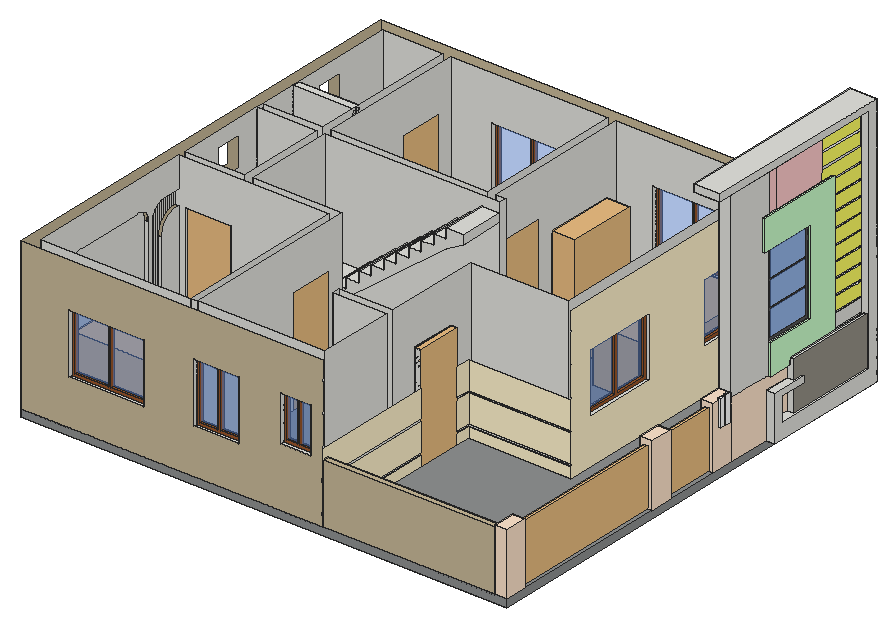
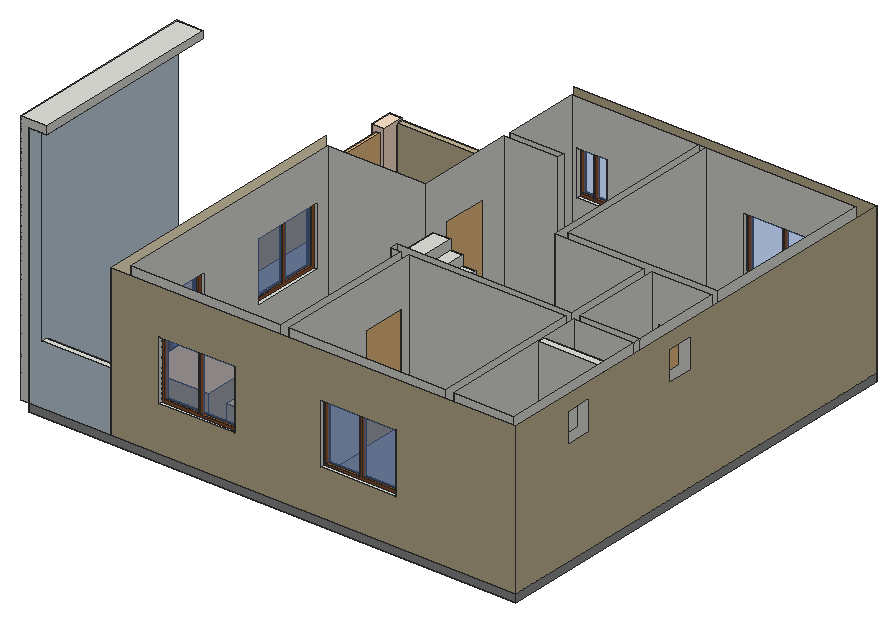
# SketchUp Ruby script. Lengths in inches.
U = 1.inch
M = Sketchup.active_model
def pt(a) = Geom::Point3d.new(a.map { |v| v * U })
def face(e, loops, mat)
  f = e.add_face(loops[0].map { |a| pt(a) })
  loops[1..].each { |l| e.add_face(l.map { |a| pt(a) }).erase! }
  f.material = f.back_material = mat if mat
  f
end
# faces: each face lists its corners as indices into pts; further lists are holes
def faces(e, pts, list, mat = nil) = list.each { |f| face(e, (f[0].is_a?(Array) ? f : [f]).map { |l| l.map { |i| pts[i] } }, mat) }
# xy, xz, yz: faces in a plane at the given z, y or x. An outline is a flat list of corners, or four numbers for a rectangle; further outlines are holes
def ring(l) = l.size == 4 ? [[l[0], l[1]], [l[2], l[1]], [l[2], l[3]], [l[0], l[3]]] : l.each_slice(2).to_a
def flat(e, list, mat, &to3) = list.each { |f| face(e, (f[0].is_a?(Array) ? f : [f]).map { |l| ring(l).map { |u, v| to3.(u, v) } }, mat) }
def xy(e, z, list, mat = nil) = flat(e, list, mat) { |x, y| [x, y, z] }
def xz(e, y, list, mat = nil) = flat(e, list, mat) { |x, z| [x, y, z] }
def yz(e, x, list, mat = nil) = flat(e, list, mat) { |y, z| [x, y, z] }
def lines(e, pts, list) = list.each { |a, b| e.add_line(pt(pts[a]), pt(pts[b])) }
# prism: a flat outline (further loops are holes) pulled along v
def prism(e, loops, v, mat = nil)
  f = face(e, loops, mat); d = Geom::Vector3d.new(v.map { |x| x * U })
  f.pushpull(f.normal.samedirection?(d) ? d.length : -d.length)
end
def box(e, o, s, mat = nil) = prism(e, [[o, [o[0] + s[0], o[1], o[2]], [o[0] + s[0], o[1] + s[1], o[2]], [o[0], o[1] + s[1], o[2]]]], [0, 0, s[2]], mat)
def at(x, y, z, deg = 0) = Geom::Transformation.translation(pt([x, y, z])) * Geom::Transformation.rotation(ORIGIN, Z_AXIS, deg.degrees)
def axes(o, x, y, z) = Geom::Transformation.new([*x, 0, *y, 0, *z, 0, *pt(o).to_a, 1])
def part(name) = M.definitions.add(name)
# library, detail: a bought-in or finely detailed component or shape, given as its bounding box
def library(name, o, s) = part(name).tap { |d| box(d.entities, o, s) }
def detail(e, o, s) = box(e.add_group.entities, o, s)
def put(e, d, t, mat = nil) = e.add_instance(d, t).tap { |i| i.material = mat if mat }
def group(e, t, mat = nil) = e.add_group.tap { |g| g.transformation = t; g.material = mat if mat }.entities
root = M.entities
M.materials.add("[Blacktop Old 02]").color = [143, 145, 145]
M.materials.add("[Color A01]").color = [255, 204, 204]
M.materials.add("[Color C01]").color = [255, 229, 204]
M.materials.add("[Color D01]").color = [255, 242, 204]
M.materials.add("[Color E03]").color = [255, 255, 101]
M.materials.add("[Color F02]").color = [204, 255, 153]
M.materials.add("[Color G01]").color = [204, 255, 204]
M.materials.add("[Color M00]").color = [255, 255, 255]
M.materials.add("[Color M06]").color = [86, 86, 86]
M.materials.add("[Formica Graystone]").color = [149, 146, 135]
M.materials.add("[Quartz Light Brown]").color = [199, 184, 152]
M.materials.add("[Terrazzo Light Blue]").color = [196, 214, 227]
M.materials.add("[Translucent Glass Blue]").color = [100, 149, 237]
M.materials["[Translucent Glass Blue]"].alpha = 0.5
M.materials.add("[Wood Cherry Original]").color = [152, 86, 42]
c1 = library("Untitled",[0,0,0],[36,4.39,84])
c2 = library("BED 3",[-244.73,-59.6875,196.6875],[91.01,69.4,39.64])
c3 = part("Group238\#1")
xy(c3.entities,0,[[732.96,223.85,732.96,355,677.96,355,677.96,360,737.96,360,737.96,223.85],[737.96,223.85,737.96,360,742.96,360,742.96,352.78,749.96,352.78,749.96,258.85,742.96,258.85,742.96,223.85],[742.96,352.78,749.96,360]])
xy(c3.entities,12.5,[[742.96,265.41,749.96,265.41,749.96,352.78,747.96,352.78,747.96,279.6,742.96,279.6]])
xy(c3.entities,31.3125,[[742.96,265.41,742.96,279.6,747.96,279.6,747.96,287.78,749.96,287.78,749.96,265.41],[742.96,279.6,747.96,287.78]])
xy(c3.entities,36,[[742.96,258.85,749.96,258.85,749.96,287.78,747.96,287.78,747.96,279.6,742.96,279.6],[742.96,279.6,747.96,287.78]])
xy(c3.entities,45.67,[[742.96,279.6,745.4,324.53],[742.96,324.53,745.4,352.78]])
xy(c3.entities,45.67,[[742.96,260.66,745.4,279.6]],"[Color G01]")
xy(c3.entities,48,[[677.96,355,732.96,360]])
xy(c3.entities,48.71,[[741.96,323.53,742.96,324.53,742.96,352.78,741.96,352.78]])
xy(c3.entities,50.65,[[741.96,323.53,741.96,352.78,742.96,352.78,742.96,324.53]])
xy(c3.entities,50.99,[[745.4,279.6,747.96,352.78]])
xy(c3.entities,60.71,[[741.96,323.53,742.96,324.53,742.96,352.78,741.96,352.78]])
xy(c3.entities,62.65,[[741.96,323.53,741.96,352.78,742.96,352.78,742.96,324.53]])
xy(c3.entities,69.67,[[742.96,260.66,745.4,300.53]],"[Color G01]")
xy(c3.entities,72.71,[[741.96,323.53,742.96,324.53,742.96,352.78,741.96,352.78]])
xy(c3.entities,74.65,[[741.96,323.53,741.96,352.78,742.96,352.78,742.96,324.53]])
xy(c3.entities,84.71,[[741.96,323.53,742.96,324.53,742.96,352.78,741.96,352.78]])
xy(c3.entities,86.65,[[741.96,323.53,741.96,352.78,742.96,352.78,742.96,324.53]])
xy(c3.entities,96.71,[[741.96,323.53,742.96,324.53,742.96,352.78,741.96,352.78]])
xy(c3.entities,98.65,[[741.96,323.53,741.96,352.78,742.96,352.78,742.96,324.53]])
xy(c3.entities,108.71,[[741.96,323.53,742.96,324.53,742.96,352.78,741.96,352.78]])
xy(c3.entities,110.65,[[741.96,323.53,741.96,352.78,742.96,352.78,742.96,324.53]])
xy(c3.entities,120.71,[[741.96,323.53,742.96,324.53,742.96,352.78,741.96,352.78]])
xy(c3.entities,122.65,[[741.96,323.53,741.96,352.78,742.96,352.78,742.96,324.53]])
xy(c3.entities,132.71,[[741.96,323.53,742.96,324.53,742.96,352.78,741.96,352.78]])
xy(c3.entities,134.65,[[741.96,323.53,741.96,352.78,742.96,352.78,742.96,324.53]])
xy(c3.entities,137.1875,[[742.96,254.35,745.4,300.53]],"[Color F02]")
xy(c3.entities,144.71,[[741.96,323.53,742.96,324.53,742.96,352.78,741.96,352.78]])
xy(c3.entities,146.65,[[741.96,323.53,741.96,352.78,742.96,352.78,742.96,324.53]])
xy(c3.entities,156.71,[[741.96,323.53,742.96,324.53,742.96,352.78,741.96,352.78]])
xy(c3.entities,158.65,[[741.96,323.53,741.96,352.78,742.96,352.78,742.96,324.53]])
xy(c3.entities,161.1875,[[742.96,254.35,745.4,324.53]],"[Color G01]")
xy(c3.entities,168.71,[[741.96,314.62,742.96,352.78]])
xy(c3.entities,170.65,[[741.96,314.62,742.96,352.78]])
xy(c3.entities,180.71,[[741.96,314.62,742.96,352.78]])
xy(c3.entities,182.65,[[741.96,314.62,742.96,352.78]])
xy(c3.entities,192.71,[[741.96,314.62,742.96,352.78]])
xy(c3.entities,194.65,[[741.96,314.62,742.96,352.78]])
xy(c3.entities,197.1875,[[729.15,203.85,732.96,360],[732.96,203.85,742.96,223.85],[742.96,203.85,749.96,269.23],[732.96,223.85,742.96,360],[742.96,269.23,749.96,314.62],
  [742.96,314.62,749.96,352.78]])
xy(c3.entities,203,[[729.15,203.85,749.96,360]])
xz(c3.entities,203.85,[[729.15,197.1875,749.96,203]])
xz(c3.entities,223.85,[[737.96,0,742.96,0,742.96,197.1875,732.96,197.1875,732.96,48,737.96,48]])
xz(c3.entities,254.35,[[742.96,137.1875,745.4,161.1875]],"[Color G01]")
xz(c3.entities,258.85,[[742.96,0,749.96,36]])
xz(c3.entities,260.66,[[742.96,45.67,745.4,69.67]],"[Color G01]")
xz(c3.entities,265.41,[[742.96,12.5,749.96,31.3125]])
xz(c3.entities,279.6,[[742.96,12.5,747.96,31.3125],[742.96,36,747.96,36,747.96,50.99,745.4,50.99,745.4,45.67,742.96,45.67]])
xz(c3.entities,287.78,[[742.96,31.3125,747.96,36],[747.96,31.3125,749.96,36]])
xz(c3.entities,300.53,[[742.96,69.67,745.4,137.1875]],"[Color G01]")
xz(c3.entities,314.62,[[741.96,168.71,742.96,170.65],[741.96,180.71,742.96,182.65],[741.96,192.71,742.96,194.65]])
xz(c3.entities,324.53,[[742.96,45.67,745.4,161.1875]],"[Color G01]")
xz(c3.entities,352.78,[[742.96,12.5,747.96,45.67],[747.96,12.5,749.96,12.5,749.96,197.1875,742.96,197.1875,742.96,45.67,745.4,45.67,745.4,50.99,747.96,50.99]])
xz(c3.entities,355,[[677.96,0,732.96,48]],"[Terrazzo Light Blue]")
xz(c3.entities,360,[[742.96,0,742.96,197.1875,729.15,197.1875,729.15,203,749.96,203,749.96,0]])
xz(c3.entities,360,[[677.96,0,677.96,48,732.96,48,732.96,197.1875,742.96,197.1875,742.96,0]],"[Terrazzo Light Blue]")
yz(c3.entities,677.96,[[355,0,360,48]])
yz(c3.entities,729.15,[[203.85,197.1875,360,203]])
yz(c3.entities,732.96,[[223.85,0,223.85,197.1875,360,197.1875,360,48,355,48,355,0]],"[Terrazzo Light Blue]")
yz(c3.entities,741.96,[[323.53,48.71,352.78,50.65],[323.53,60.71,352.78,62.65],[323.53,72.71,352.78,74.65],[323.53,84.71,352.78,86.65],[323.53,96.71,352.78,98.65],
  [323.53,108.71,352.78,110.65],[323.53,120.71,352.78,122.65],[323.53,132.71,352.78,134.65],[323.53,144.71,352.78,146.65],[323.53,156.71,352.78,158.65],
  [314.62,168.71,352.78,170.65],[314.62,180.71,352.78,182.65],[314.62,192.71,352.78,194.65]])
yz(c3.entities,742.96,[[352.78,0,360,45.67],[265.41,31.3125,265.41,32.125,258.85,32.125,258.85,36,279.6,36,279.6,31.3125],[279.6,31.3125,287.78,36],[223.85,45.67,260.66,45.67,260.66,137.1875,254.35,137.1875,254.35,161.1875,261.79,161.1875,261.79,197.1875,223.85,197.1875],[260.66,45.67,260.66,69.67,300.53,69.67,300.53,137.1875,254.35,137.1875,254.35,161.1875,324.53,161.1875,324.53,45.67],
  [324.53,45.67,352.78,48.71],[352.78,45.67,360,197.1875],[324.53,50.65,352.78,60.71],[314.62,168.71,352.78,170.65],[314.62,192.71,352.78,194.65]])
yz(c3.entities,742.96,[[261.79,161.1875,269.23,197.1875],[269.23,161.1875,314.62,197.1875]],"[Color A01]")
yz(c3.entities,742.96,[[223.85,0,258.85,0,258.85,36,279.6,36,279.6,45.67,223.85,45.67],[265.41,12.5,279.6,31.3125]],"[Color C01]")
yz(c3.entities,742.96,[[324.53,62.65,352.78,72.71],[324.53,74.65,352.78,84.71],[324.53,86.65,352.78,96.71],[324.53,98.65,352.78,108.71],[324.53,110.65,352.78,120.71],
  [324.53,122.65,352.78,132.71],[324.53,134.65,352.78,144.71],[324.53,146.65,352.78,156.71],[324.53,158.65,352.78,158.65,352.78,168.71,314.62,168.71,314.62,161.1875,324.53,161.1875],[314.62,170.65,352.78,180.71],
  [314.62,182.65,352.78,192.71],[314.62,194.65,352.78,197.1875]],"[Color E03]")
yz(c3.entities,742.96,[[314.62,180.71,352.78,182.65]],"[Color M00]")
yz(c3.entities,742.96,[[[260.66,69.67,300.53,137.1875],[262.66,71.67,298.53,92.49],[262.66,114.37,298.53,135.1875],[262.66,93.2,298.53,113.66]]],"[Color M06]")
yz(c3.entities,742.96,[[262.66,71.67,298.53,92.49],[262.66,93.2,298.53,113.66],[262.66,114.37,298.53,135.1875]],"[Translucent Glass Blue]")
yz(c3.entities,745.4,[[279.6,45.67,324.53,50.99],[324.53,45.67,352.78,50.99]])
yz(c3.entities,745.4,[[260.66,45.67,279.6,45.67,279.6,50.99,324.53,50.99,324.53,161.1875,254.35,161.1875,254.35,137.1875,300.53,137.1875,300.53,69.67,260.66,69.67]],"[Color G01]")
yz(c3.entities,747.96,[[279.6,12.5,352.78,12.5,352.78,50.99,279.6,50.99,279.6,36,287.78,36,287.78,31.3125,279.6,31.3125]],"[Formica Graystone]")
yz(c3.entities,749.96,[[258.85,0,360,0,360,203,203.85,203,203.85,197.1875,352.78,197.1875,352.78,12.5,265.41,12.5,265.41,31.3125,287.78,31.3125,287.78,36,258.85,36]])
p = [[742.96,265.41,0],[742.96,265.41,12.5]]
lines(c3.entities,p,[[0,1]])
g1 = group(c3.entities,at(732.96,223.85,0),"[Color C01]")
box(g1,[0,-18,0],[10,18,49.5625])
box(g1,[0,-78.85,0],[10,18,49.5625])
box(g1,[0,-223.85,0],[10,18,49.5625])
g2 = group(g1,at(10,-13.38,30.8125),"[Color M00]")
box(g2,[0,0,0],[2,3.5625,21])
g3 = group(g1,at(10,-7.63,30.8125),"[Color M00]")
box(g3,[0,0,0],[2,3.5625,21])
c4 = library("Vask",[0,0,0],[10.95,18.9,37.68])
c5 = library("CS300DRT",[0,0,0],[27.18,17.85,30.31])
c6 = library("sofa blue",[10.44,18.33,0.01],[94.56,54.06,43.33])
c7 = library("Metal Gate",[-307.875,157.48,0],[187.84,3,45.27])
c8 = library("Group\#10",[0,0,0],[54.56,69.25,18.34])
c9 = part("Group222\#1")
prism(c9.entities,[[[-13.5,36,0],[-13.5,48,0],[-12,48,0],[-12,36.07,0]]],[0,0,0.6875])
c10 = part("Group223\#1")
xy(c10.entities,0,[[-10,35.97,-11.36,36.1,-11.5,36.09,-11.5,48,-10,48]])
xy(c10.entities,0.6875,[[-10,35.97,-10,48,-11.5,48,-11.5,36.09,-11.36,36.1]])
xz(c10.entities,48,[[-11.5,0,-10,0.6875]])
yz(c10.entities,-11.5,[[36.09,0,48,0.6875]])
yz(c10.entities,-10,[[35.97,0,48,0.6875]])
c11 = part("Group224\#1")
xy(c11.entities,0,[[-8,35.61,-9.23,35.9,-9.5,35.93,-9.5,48,-8,48]])
xy(c11.entities,0.6875,[[-8,35.61,-8,48,-9.5,48,-9.5,35.93,-9.23,35.9]])
xz(c11.entities,48,[[-9.5,0,-8,0.6875]])
yz(c11.entities,-9.5,[[35.93,0,48,0.6875]])
yz(c11.entities,-8,[[35.61,0,48,0.6875]])
c12 = part("Group225\#1")
xy(c12.entities,0,[[-6,34.95,-7.15,35.41,-7.5,35.49,-7.5,48,-6,48]])
xy(c12.entities,0.6875,[[-6,34.95,-6,48,-7.5,48,-7.5,35.49,-7.15,35.41]])
xz(c12.entities,48,[[-7.5,0,-6,0.6875]])
yz(c12.entities,-7.5,[[35.49,0,48,0.6875]])
yz(c12.entities,-6,[[34.95,0,48,0.6875]])
c13 = part("Group226\#1")
xy(c13.entities,0,[[-4,33.96,-5.16,34.625,-5.5,34.76,-5.5,48,-4,48]])
xy(c13.entities,0.6875,[[-4,33.96,-4,48,-5.5,48,-5.5,34.76,-5.16,34.625]])
xz(c13.entities,48,[[-5.5,0,-4,0.6875]])
yz(c13.entities,-5.5,[[34.76,0,48,0.6875]])
yz(c13.entities,-4,[[33.96,0,48,0.6875]])
c14 = part("Group227\#1")
xy(c14.entities,0,[[-2,32.57,-3.3,33.57,-3.5,33.68,-3.5,48,-2,48]])
xy(c14.entities,0.6875,[[-2,32.57,-2,48,-3.5,48,-3.5,33.68,-3.3,33.57]])
yz(c14.entities,-3.5,[[33.68,0,48,0.6875]])
yz(c14.entities,-2,[[32.57,0,48,0.6875]])
c15 = part("Group228\#1")
xy(c15.entities,0,[[0,30.58,-0.11,30.74,-1.5,32.15,-1.5,48,0,48]])
xy(c15.entities,0.6875,[[0,30.58,0,48,-1.5,48,-1.5,32.15,-0.11,30.74]])
xz(c15.entities,48,[[-1.5,0,0,0.6875]])
yz(c15.entities,-1.5,[[32.15,0,48,0.6875]])
yz(c15.entities,0,[[30.58,0,48,0.6875]])
c16 = part("Group229\#1")
xy(c16.entities,0,[[2,27.43,1.15,29.01,0.5,29.9,0.5,48,1.15,48,2,47.97]])
xy(c16.entities,0.6875,[[2,27.43,2,47.97,1.15,48,0.5,48,0.5,29.9,1.15,29.01]])
yz(c16.entities,0.5,[[29.9,0,48,0.6875]])
yz(c16.entities,2,[[27.43,0,47.97,0.6875]])
c17 = part("Group230\#1")
xy(c17.entities,0,[[3.5,-48,3.5,20.89,3.35,23.03,2.9,25.12,2.5,26.21,2.5,47.95,2.75,47.9375,4,47.72,4,-48]])
xy(c17.entities,0.6875,[[3.5,-48,4,-48,4,47.72,2.75,47.9375,2.5,47.95,2.5,26.21,2.9,25.12,3.35,23.03,3.5,20.89]])
yz(c17.entities,2.5,[[26.21,0,47.95,0.6875]])
yz(c17.entities,4,[[-48,0,47.72,0.6875]])
c18 = part("Group231\#1")
xy(c18.entities,0,[[4.5,-48,4.5,47.61,5.85,47.1875,6,47.12,6,-48]])
xy(c18.entities,0.6875,[[4.5,-48,6,-48,6,47.12,5.85,47.1875,4.5,47.61]])
xz(c18.entities,-48,[[4.5,0,6,0.6875]])
yz(c18.entities,4.5,[[-48,0,47.61,0.6875]])
yz(c18.entities,6,[[-48,0,47.12,0.6875]])
c19 = part("Group232\#1")
xy(c19.entities,0,[[6.5,-48,6.5,46.88,7.3,46.51,8,46.06,8,-48]])
xy(c19.entities,0.6875,[[6.5,-48,8,-48,8,46.06,7.3,46.51,6.5,46.88]])
xz(c19.entities,-48,[[6.5,0,8,0.6875]])
yz(c19.entities,6.5,[[-48,0,46.88,0.6875]])
yz(c19.entities,8,[[-48,0,46.06,0.6875]])
c20 = part("Group233\#1")
xy(c20.entities,0,[[8.5,-48,8.5,45.74,8.64,45.64,9.86,44.61,10,44.46,10,-48]])
xy(c20.entities,0.6875,[[8.5,-48,10,-48,10,44.46,9.86,44.61,8.64,45.64,8.5,45.74]])
xz(c20.entities,-48,[[8.5,0,10,0.6875]])
yz(c20.entities,8.5,[[-48,0,45.74,0.6875]])
yz(c20.entities,10,[[-48,0,44.46,0.6875]])
c21 = part("Group234\#1")
xy(c21.entities,0,[[10.5,-48,10.5,43.9,10.93,43.42,11.83,42.1,12,41.77,12,-48]])
xy(c21.entities,0.6875,[[10.5,-48,12,-48,12,41.77,11.83,42.1,10.93,43.42,10.5,43.9]])
xz(c21.entities,-48,[[10.5,0,12,0.6875]])
yz(c21.entities,10.5,[[-48,0,43.9,0.6875]])
yz(c21.entities,12,[[-48,0,41.77,0.6875]])
c22 = part("Group235\#1")
xy(c22.entities,0,[[12.5,-48,12.5,40.78,12.55,40.67,13.08,39.16,13.39,37.6,13.5,36,13.5,-48]])
xy(c22.entities,0.6875,[[12.5,-48,13.5,-48,13.5,36,13.39,37.6,13.08,39.16,12.55,40.67,12.5,40.78]])
yz(c22.entities,12.5,[[-48,0,40.78,0.6875]])
c23 = part("Group220\#1")
put(c23.entities,c9,at(0,0,0))
put(c23.entities,c10,at(0,0,0))
put(c23.entities,c11,at(0,0,0))
put(c23.entities,c12,at(0,0,0))
put(c23.entities,c13,at(0,0,0))
put(c23.entities,c14,at(0,0,0))
put(c23.entities,c15,at(0,0,0))
put(c23.entities,c16,at(0,0,0))
put(c23.entities,c17,at(0,0,0))
put(c23.entities,c18,at(0,0,0))
put(c23.entities,c19,at(0,0,0))
put(c23.entities,c20,at(0,0,0))
put(c23.entities,c21,at(0,0,0))
put(c23.entities,c22,at(0,0,0))
c24 = part("Group236\#1")
box(c24.entities,[595.96,0,0],[137,5,48],"[Quartz Light Brown]")
c25 = library("Porada+-+Icaro+Table",[-0.02,6.95,0.04],[51.6,51.6,29.59])
c26 = library("1-POIGNEE CLC2",[-3.03,-0.375,0],[6.06,0.75,1.42])
c27 = part("Group7\#2")
xy(c27.entities,0,[[-28,-22,-1,22],[1,-22,28,22]])
c28 = part("Group6\#1")
prism(c28.entities,[[[-30,24,0],[30,24,0],[30,-24,0],[-30,-24,0]],[[1,-22,0],[28,-22,0],[28,22,0],[1,22,0]],[[-28,-22,0],[-1,-22,0],[-1,22,0],[-28,22,0]]],[0,0,3])
put(c28.entities,c27,at(0,0,1.5),"[Translucent Glass Blue]")
c29 = part("Group9\#2")
xy(c29.entities,0,[[-16,-22,-1,22],[1,-22,16,22]])
c30 = part("Group8\#1")
prism(c30.entities,[[[18,24,0],[18,-24,0],[-18,-24,0],[-18,24,0]],[[-16,-22,0],[-1,-22,0],[-1,22,0],[-16,22,0]],[[1,-22,0],[16,-22,0],[16,22,0],[1,22,0]]],[0,0,3])
put(c30.entities,c29,at(0,0,1.5),"[Translucent Glass Blue]")
c31 = part("Group13\#2")
xy(c31.entities,0,[[-28,-22,-1,22],[1,-22,28,22]])
c32 = part("Group12\#1")
prism(c32.entities,[[[30,-24,0],[-30,-24,0],[-30,24,0],[30,24,0]],[[-1,22,0],[-28,22,0],[-28,-22,0],[-1,-22,0]],[[28,-22,0],[28,22,0],[1,22,0],[1,-22,0]]],[0,0,3])
put(c32.entities,c31,at(0,0,1.5),"[Translucent Glass Blue]")
c33 = part("Group15\#2")
xy(c33.entities,0,[[-28,-22,-1,22],[1,-22,28,22]])
c34 = part("Group14\#1")
prism(c34.entities,[[[-30,-24,0],[-30,24,0],[30,24,0],[30,-24,0]],[[-1,22,0],[-28,22,0],[-28,-22,0],[-1,-22,0]],[[1,-22,0],[28,-22,0],[28,22,0],[1,22,0]]],[0,0,3])
put(c34.entities,c33,at(0,0,1.5),"[Translucent Glass Blue]")
c35 = part("Group17\#2")
xy(c35.entities,0,[[-28,-22,-1,22],[1,-22,28,22]])
c36 = part("Group16\#1")
prism(c36.entities,[[[-30,-24,0],[-30,24,0],[30,24,0],[30,-24,0]],[[-1,22,0],[-28,22,0],[-28,-22,0],[-1,-22,0]],[[28,-22,0],[28,22,0],[1,22,0],[1,-22,0]]],[0,0,3])
put(c36.entities,c35,at(0,0,1.5),"[Translucent Glass Blue]")
c37 = part("Group19\#2")
xy(c37.entities,0,[[-28,-22,-1,22],[1,-22,28,22]])
c38 = part("Group18\#1")
prism(c38.entities,[[[-30,-24,0],[-30,24,0],[30,24,0],[30,-24,0]],[[1,22,0],[1,-22,0],[28,-22,0],[28,22,0]],[[-1,22,0],[-28,22,0],[-28,-22,0],[-1,-22,0]]],[0,0,3])
put(c38.entities,c37,at(0,0,1.5),"[Translucent Glass Blue]")
c39 = library("download?mid=50c7180b9fccec56d493bfe20f94b6ab&ctyp=sp&cv=p8.",[149.43,43.83,17.86],[74.75,0.57,42.04])
c40 = part("Group11\#2")
xy(c40.entities,0,[[-10,-16,-1,16],[1,-16,10,16]])
c41 = part("Group10\#1")
prism(c41.entities,[[[12,-18,0],[-12,-18,0],[-12,18,0],[12,18,0]],[[-1,16,0],[-10,16,0],[-10,-16,0],[-1,-16,0]],[[1,16,0],[1,-16,0],[10,-16,0],[10,16,0]]],[0,0,3])
put(c41.entities,c40,at(0,0,1.5),"[Translucent Glass Blue]")
xy(root,0,[[0,36,0,396,324,396,324,181,242,181,242,169.9,236.5,169.9,236.5,190,315,190,315,387,195,387,195,310.07,189,310.07,189,387,63,387,63,375.41,57,375.41,57,387,9,387,9,189,15,189,15,183,9,183,9,166,5.25,166,5.25,156,9,156,9,153,5.25,153,5.25,75,9,75,9,72,5.25,72,5.25,62,9,62,9,45,236.5,45,236.5,105.96,193.6875,105.96,193.6875,111.96,236.5,111.96,236.5,133.9,242,133.9,242,36],[0,36,39,36,39,45,9,45,9,387,96,387,96,396,0,396],[208.27,36,232.27,45],[129,45,134.5,140.13],[236.5,169.9,242,169.9,242,181,324,181,324,199.85,315,199.85,315,190,236.5,190],
  [129,176.13,129,183,51,183,51,189,134.5,189,134.5,176.13],[57,189,57,261,9,261,9,267,189,267,189,274.07,195,274.07,195,267,202.86,267,202.86,261,63,261,63,189],[9,261,202.86,261,202.86,267,195,267,195,274.07,189,274.07,189,267,9,267],[57,267,63,339.41],[57,267,63,339.41],
  [57,375.41,63,387]])
xy(root,8.32,[[241,36,242,133.9],[241,169.9,242,169.9,242,181,241,182],[242,181,324,181,324,182,241,182]])
xy(root,10.26,[[241,36,242,133.9],[241,169.9,241,182,242,181,242,169.9],[242,181,241,182,324,182,324,181]])
xy(root,32.32,[[241,36,242,133.9],[241,169.9,242,169.9,242,181,241,182],[242,181,324,181,324,182,241,182]])
xy(root,34.26,[[241,36,242,133.9],[241,169.9,241,182,242,181,242,169.9],[242,181,241,182,324,182,324,181]])
xy(root,36,[[39,36,99,45],[138.68,36,174.68,45],[315,199.85,324,259.85],[315,313.375,324,373.375],[96,387,156,396],
  [225,387,285,396]])
xy(root,48,[[208.27,36,232.27,45]])
xy(root,120,[[9,297,57,303]])
xz(root,36,[[241,8.32,242,10.26],[241,32.32,242,34.26]])
xz(root,36,[[[0,0,242,0,242,8.32,241,8.32,241,10.26,242,10.26,242,32.32,241,32.32,241,34.26,242,34.26,242,56.32,241,56.32,241,58.26,242,58.26,242,80.32,241,80.32,241,82.26,242,82.26,242,104.32,241,104.32,241,106.26,242,106.26,242,120,0,120],[39,36,99,84],[138.68,36,174.68,84],[208.27,48,232.27,84]]],"[Quartz Light Brown]")
xz(root,45,[[[9,0,9,84,5.25,84,5.25,96,9,96,9,120,129,120,129,0],[39,36,99,84]],[129,0,134.5,120],[[134.5,0,236.5,120],[138.68,36,174.68,84],[208.27,48,232.27,84]]])
xz(root,62,[[5.25,0,9,68.89]])
xz(root,72,[[5.25,0,9,84]])
xz(root,75,[[5.25,0,9,85.6]])
xz(root,105.96,[[193.6875,0,236.5,120]])
xz(root,111.96,[[193.6875,0,236.5,120]])
xz(root,133.9,[[236.5,0,236.5,84,242,84,242,82.26,241,82.26,241,80.32,242,80.32,242,58.26,241,58.26,241,56.32,242,56.32,242,34.26,241,34.26,241,32.32,242,32.32,242,10.26,241,10.26,241,8.32,242,8.32,242,0],[241,8.32,242,10.26],[241,32.32,242,34.26]])
xz(root,140.13,[[129,0,134.5,84]])
xz(root,153,[[5.25,0,9,85.6]])
xz(root,156,[[5.25,0,9,84]])
xz(root,166,[[5.25,0,9,68.89]])
xz(root,169.9,[[236.5,0,242,0,242,8.32,241,8.32,241,10.26,242,10.26,242,32.32,241,32.32,241,34.26,242,34.26,242,56.32,241,56.32,241,58.26,242,58.26,242,80.32,241,80.32,241,82.26,242,82.26,242,84,236.5,84],[241,8.32,242,10.26],[241,32.32,242,34.26]])
xz(root,176.13,[[129,0,134.5,84]])
xz(root,181,[[242,0,324,8.32],[242,10.26,324,32.32],[242,34.26,324,56.32]],"[Color D01]")
xz(root,182,[[241,8.32,324,10.26],[241,32.32,324,34.26]])
xz(root,183,[[9,0,15,0,15,84,51,84,51,0,129,0,129,120,9,120,9,96,5.25,96,5.25,84,9,84]])
xz(root,189,[[9,0,9,120,57,120,57,0,51,0,51,84,15,84,15,0],[63,0,134.5,120]])
xz(root,190,[[236.5,0,315,120]])
xz(root,199.85,[[315,36,324,84]])
xz(root,259.85,[[315,36,324,84]])
xz(root,261,[[9,0,57,120],[63,0,202.86,120]])
xz(root,267,[[9,0,57,120],[63,0,189,120],[195,0,202.86,120]])
xz(root,274.07,[[189,0,195,84]])
xz(root,297,[[9,0,57,120]])
xz(root,303,[[9,0,57,120]])
xz(root,310.07,[[189,0,195,84]])
xz(root,313.375,[[315,36,324,84]])
xz(root,339.41,[[57,0,63,84]])
xz(root,373.375,[[315,36,324,84]])
xz(root,375.41,[[57,0,63,84]])
xz(root,387,[[9,0,57,120],[[63,0,189,120],[96,36,156,84]],[[195,0,315,120],[225,36,285,84]]])
xz(root,396,[[[0,0,324,120],[225,36,285,84],[96,36,156,84]]],"[Quartz Light Brown]")
yz(root,0,[[[36,0,396,120],[221.625,84,243.48,108],[322.71,84,344.375,108]]],"[Quartz Light Brown]")
yz(root,5.25,[[75,0,153,0,153,85.6,152.97,87.12,152.71,88.62,152.23,90.07,151.53,91.42,150.63,92.65,149.56,93.73,148.33,94.64,146.98,95.34,145.54,95.84,144.04,96.1,142.51,96.14,141,95.9375,87,95.9375,85.49,96.14,83.96,96.1,82.46,95.84,81.02,95.34,79.67,94.64,78.44,93.73,77.37,92.65,76.47,91.42,75.77,90.07,75.29,88.62,75.03,87.12,75,85.6],[156,0,166,0,166,68.89,166.15,71.03,166.6,73.12,167.34,75.125,168.35,77.01,169.61,78.74,171.11,80.26,172.8,81.57,174.66,82.625,176.65,83.41,178.73,83.9,180.86,84.1,183,84,183,96,168.35,96,166.75,95.9375,165.17,95.67,163.65,95.1875,162.2,94.51,160.86,93.64,159.64,92.61,158.57,91.42,157.67,90.1,156.95,88.67,156.42,87.16,156.11,85.6,156,84]])
yz(root,9,[[45,0,62,0,62,68.89,61.85,71.03,61.4,73.12,60.66,75.125,59.65,77.01,58.39,78.74,56.89,80.26,55.2,81.57,53.34,82.625,51.35,83.41,49.27,83.9,47.14,84.1,45,84],[72,0,75,0,75,85.6,75.03,87.12,75.29,88.62,75.77,90.07,76.47,91.42,77.37,92.65,78.44,93.73,79.67,94.64,81.02,95.34,82.46,95.84,83.96,96.1,85.49,96.14,87,95.9375,141,95.9375,142.51,96.14,144.04,96.1,145.54,95.84,146.98,95.34,148.33,94.64,149.56,93.73,150.63,92.65,151.53,91.42,152.23,90.07,152.71,88.62,152.97,87.12,153,85.6,153,0,156,0,156,84,156.11,85.6,156.42,87.16,156.95,88.67,157.67,90.1,158.57,91.42,159.64,92.61,160.86,93.64,162.2,94.51,163.65,95.1875,165.17,95.67,166.75,95.9375,168.35,96,183,96,183,120,45,120,45,96,59.65,96,61.25,95.9375,62.83,95.67,64.35,95.1875,65.8,94.51,67.14,93.64,68.36,92.61,69.43,91.42,70.33,90.1,71.05,88.67,71.58,87.16,71.89,85.6,72,84],[166,0,183,0,183,84,180.86,84.1,178.73,83.9,176.65,83.41,174.66,82.625,172.8,81.57,171.11,80.26,169.61,78.74,168.35,77.01,167.34,75.125,166.6,73.12,166.15,71.03,166,68.89],[[189,0,261,120],[221.625,84,243.48,108]],[261,0,267,120],
  [[267,0,387,120],[322.71,84,344.375,108]],[297,0,303,120]])
yz(root,15,[[183,0,189,84]])
yz(root,39,[[36,36,45,84]])
yz(root,51,[[183,0,189,84]])
yz(root,57,[[189,0,261,120],[267,0,267,120,387,120,387,0,375.41,0,375.41,84,339.41,84,339.41,0],[297,0,303,120]])
yz(root,63,[[189,0,261,120],[267,0,339.41,0,339.41,84,375.41,84,375.41,0,387,0,387,120,267,120]])
yz(root,96,[[387,36,396,84]])
yz(root,99,[[36,36,45,84]])
yz(root,129,[[45,0,45,120,183,120,183,0,176.13,0,176.13,84,140.13,84,140.13,0]])
yz(root,134.5,[[45,0,140.13,0,140.13,84,176.13,84,176.13,0,189,0,189,120,45,120]])
yz(root,138.68,[[36,36,45,84]])
yz(root,156,[[387,36,396,84]])
yz(root,174.68,[[36,36,45,84]])
yz(root,189,[[267,0,267,120,387,120,387,0,310.07,0,310.07,84,274.07,84,274.07,0]])
yz(root,193.6875,[[105.96,0,111.96,120]])
yz(root,195,[[267,0,274.07,0,274.07,84,310.07,84,310.07,0,387,0,387,120,267,120]])
yz(root,202.86,[[261,0,267,120]])
yz(root,208.27,[[36,48,45,84]])
yz(root,225,[[387,36,396,84]])
yz(root,232.27,[[36,48,45,84]])
yz(root,236.5,[[45,0,105.96,120],[111.96,0,111.96,120,190,120,190,0,169.9,0,169.9,84,133.9,84,133.9,0]])
yz(root,241,[[36,8.32,133.9,10.26],[169.9,8.32,182,10.26],[36,32.32,133.9,34.26],[169.9,32.32,182,34.26]])
yz(root,242,[[36,0,133.9,8.32],[169.9,0,181,8.32],[36,10.26,133.9,32.32],[169.9,10.26,181,32.32],[36,34.26,133.9,56.32],
  [169.9,34.26,181,56.32]],"[Color D01]")
yz(root,285,[[387,36,396,84]])
yz(root,315,[[[190,0,387,120],[199.85,36,259.85,84],[313.375,36,373.375,84]]])
yz(root,324,[[[181,0,396,0,396,120,181,120,181,106.26,182,106.26,182,104.32,181,104.32,181,82.26,182,82.26,182,80.32,181,80.32,181,58.26,182,58.26,182,56.32,181,56.32,181,34.26,182,34.26,182,32.32,181,32.32,181,10.26,182,10.26,182,8.32,181,8.32],[199.85,36,259.85,84],[313.375,36,373.375,84]]],"[Color D01]")
p = [[96,390.5,0],[156,390.5,0],[96,392.5,0],[156,392.5,0],[225,390.5,0],[285,390.5,0],
  [225,392.5,0],[285,392.5,0],[189,310.07,0],[195,310.07,0],[134.5,176.13,0],[129,176.07,0],
  [134.5,140.13,0],[129,140.07,0],[63,189,0],[129,189,0],[63,261,0],[129,225,0],
  [202.86,225,0],[202.86,261,0],[39,40.5,36],[39,40.5,84],[99,40.5,84],[99,40.5,36],
  [138.68,40.5,36],[138.68,40.5,84],[174.68,40.5,84],[174.68,40.5,36],[208.27,40.5,48],[208.27,40.5,84],
  [232.27,40.5,84],[232.27,40.5,48],[319.5,199.85,84],[319.5,199.85,36],[319.5,259.85,36],[319.5,259.85,84],
  [319.5,313.375,84],[319.5,313.375,36],[319.5,373.375,36],[319.5,373.375,84],[285,391.5,36],[285,391.5,84],
  [225,391.5,84],[225,391.5,36],[156,391.5,36],[156,391.5,84],[96,391.5,84],[96,391.5,36]]
lines(root,p,[[0,1],[2,3],[4,5],[6,7],[8,9],[10,11],[12,13],[14,15],[14,16],[17,15],[18,19],[17,18],
  [20,21],[22,23],[23,20],[24,25],[26,27],[27,24],[28,29],[30,31],[31,28],[32,33],[33,34],[34,35],
  [36,37],[37,38],[38,39],[40,41],[42,43],[43,40],[44,45],[46,47],[47,44]])
g4 = group(root,at(0,36,-6),"[Blacktop Old 02]")
xy(g4,0,[[0,0,389,360]])
xy(g4,6,[[[0,0,389,360],[14.13,268.73,13.13,268.99,12.24,269.5,11.51,270.23,10.99,271.11,10.72,272.11,10.72,273.13,10.98,274.13,11.49,275.02,12.21,275.75,13.1,276.27,14.09,276.54,15.12,276.54,16.11,276.28,17.01,275.77,17.74,275.05,18.26,274.16,18.53,273.17,18.53,272.14,18.27,271.15,17.76,270.25,17.04,269.52,16.15,269.01,15.16,268.74],[13.2,216.36,12.21,216.625,11.32,217.14,10.59,217.86,10.07,218.75,9.8,219.74,9.79,220.77,10.05,221.76,10.56,222.65,11.29,223.38,12.18,223.9,13.17,224.17,14.2,224.18,15.19,223.92,16.08,223.41,16.8125,222.68,17.33,221.79,17.6,220.8,17.61,219.77,17.34,218.78,16.83,217.89,16.11,217.16,15.22,216.64,14.23,216.37]],[13.2,216.36,14.23,216.37,15.22,216.64,16.11,217.16,16.83,217.89,17.34,218.78,17.61,219.77,17.6,220.8,17.33,221.79,16.8125,222.68,16.08,223.41,15.19,223.92,14.2,224.18,13.17,224.17,12.18,223.9,11.29,223.38,10.56,222.65,10.05,221.76,9.79,220.77,9.8,219.74,10.07,218.75,10.59,217.86,11.32,217.14,12.21,216.625],[14.13,268.73,15.16,268.74,16.15,269.01,17.04,269.52,17.76,270.25,18.27,271.15,18.53,272.14,18.53,273.17,18.26,274.16,17.74,275.05,17.01,275.77,16.11,276.28,15.12,276.54,14.09,276.54,13.1,276.27,12.21,275.75,11.49,275.02,10.98,274.13,10.72,273.13,10.72,272.11,10.99,271.11,11.51,270.23,12.24,269.5,13.13,268.99]])
xz(g4,0,[[0,0,389,6]])
xz(g4,360,[[0,0,389,6]])
yz(g4,0,[[0,0,360,6]])
yz(g4,389,[[0,0,360,6]])
put(root,c1,at(134.16,140.13,0,90))
put(root,c1,at(15,183.59,0))
put(root,c1,at(194.41,274.07,0,90))
put(root,c1,at(241.66,133.9,0,90))
put(root,c1,at(62.41,339.41,0,90))
put(root,c2,axes([177.02,139.93,-196.6875],[0.68503,0,0],[0,1.03755,0],[0,0,1]))
g5 = group(root,at(63.22,189,0))
prism(g5,[[[49.68,0,24.875],[38.88,0,24.875],[38.88,0,33.16],[0,0,33.16],[0,0,17.77],[38.88,0,17.77],[60.48,0,1.18],[60.48,0,0],[71.28,0,0],[71.28,0,8.29],[60.48,0,8.29],[60.48,0,16.58],[49.68,0,16.58]]],[0,36,0])
p = [[0,0,33.16],[0,0,41.46]]
lines(g5,p,[[0,1]])
put(root,c3,at(-353.96,36,0))
put(root,c4,at(9,189,0))
put(root,c2,axes([226.49,316.9375,-196.6875],[0.66,0,0],[0,0.78,0],[0,0,1]))
put(root,c5,axes([10.5,322.125,0],[1.13,0,0],[0,1.25,0],[0,0,1]))
put(root,c5,axes([10.1875,222.125,0],[1.13,0,0],[0,1.25,0],[0,0,1]))
put(root,c4,at(9,368.1,0))
put(root,c6,at(241.92,387.66,-0.01,-90))
put(root,c7,at(542.98,361.875,0,90))
put(root,c8,axes([195,323.13,0],[0,1,0],[0,0,1],[1,0,0]),"[Wood Cherry Original]")
put(root,c23,axes([5.25,58.5,48],[0,1,0],[0,0,1],[1,0,0]))
put(root,c23,axes([5.25,169.5,48],[0,-1,0],[0,0,1],[1,0,0]))
put(root,c24,at(-353.96,36,0))
put(root,c25,axes([229.38,302.35,-0.04],[0.6888,0,0],[0,1,0],[0,0,1]))
g6 = group(root,at(213,334.9,1.42),"[Wood Cherry Original]")
box(g6,[0,-0.08,-0.08],[0.71,30.62,10.7])
put(root,c26,axes([213.71,350.6875,7.27],[0,1,0],[0,0,1],[1,0,0]))
g7 = group(root,at(213,334.9,12.66),"[Wood Cherry Original]")
box(g7,[0,-0.08,-0.08],[0.71,15.04,10.7])
g8 = group(root,at(213,350.49,12.66),"[Wood Cherry Original]")
box(g8,[0,-0.08,-0.08],[0.71,15.04,10.7])
put(root,c26,axes([213.71,342.29,17.92],[0,1,0],[0,0,1],[1,0,0]))
put(root,c26,axes([213.71,357.98,17.92],[0,1,0],[0,0,1],[1,0,0]))
g9 = group(root,at(63,225,25.23))
prism(g9,[[[126,0,87.29],[126,0,79.36],[116,0,79.36],[116,0,71.42],[106,0,71.42],[106,0,63.49],[96,0,63.49],[96,0,55.55],[86,0,55.55],[86,0,47.61],[76,0,47.61],[76,0,39.68],[66,0,39.68],[66,0,31.74],[56,0,31.74],[56,0,23.81],[46,0,23.81],[46,0,15.87],[36,0,15.87],[36,0,7.9375],[0,0,7.9375],[0,0,0],[36,0,0],[36,0,1.13],[126,0,72.56],[139.86,0,80.49],[139.86,0,87.29]]],[0,36,0])
put(root,c28,axes([69,42,60],[1,0,0],[0,0,1],[0,-1,0]),"[Wood Cherry Original]")
put(root,c30,axes([156.68,42,60],[1,0,0],[0,0,1],[0,-1,0]),"[Wood Cherry Original]")
put(root,c32,axes([318,229.85,60],[0,1,0],[0,0,1],[1,0,0]),"[Wood Cherry Original]")
put(root,c34,axes([318,343.375,60],[0,1,0],[0,0,1],[1,0,0]),"[Wood Cherry Original]")
put(root,c36,axes([255,390,60],[-1,0,0],[0,0,1],[0,1,0]),"[Wood Cherry Original]")
put(root,c38,axes([126,390,60],[-1,0,0],[0,0,1],[0,1,0]),"[Wood Cherry Original]")
put(root,c39,axes([326.87,283,30.1],[0.00269,0.35312,0],[-2.7665,0.02108,0],[0,0,0.40605]))
put(root,c41,axes([220.27,42,66],[1,0,0],[0,0,1],[0,-1,0]),"[Wood Cherry Original]")
